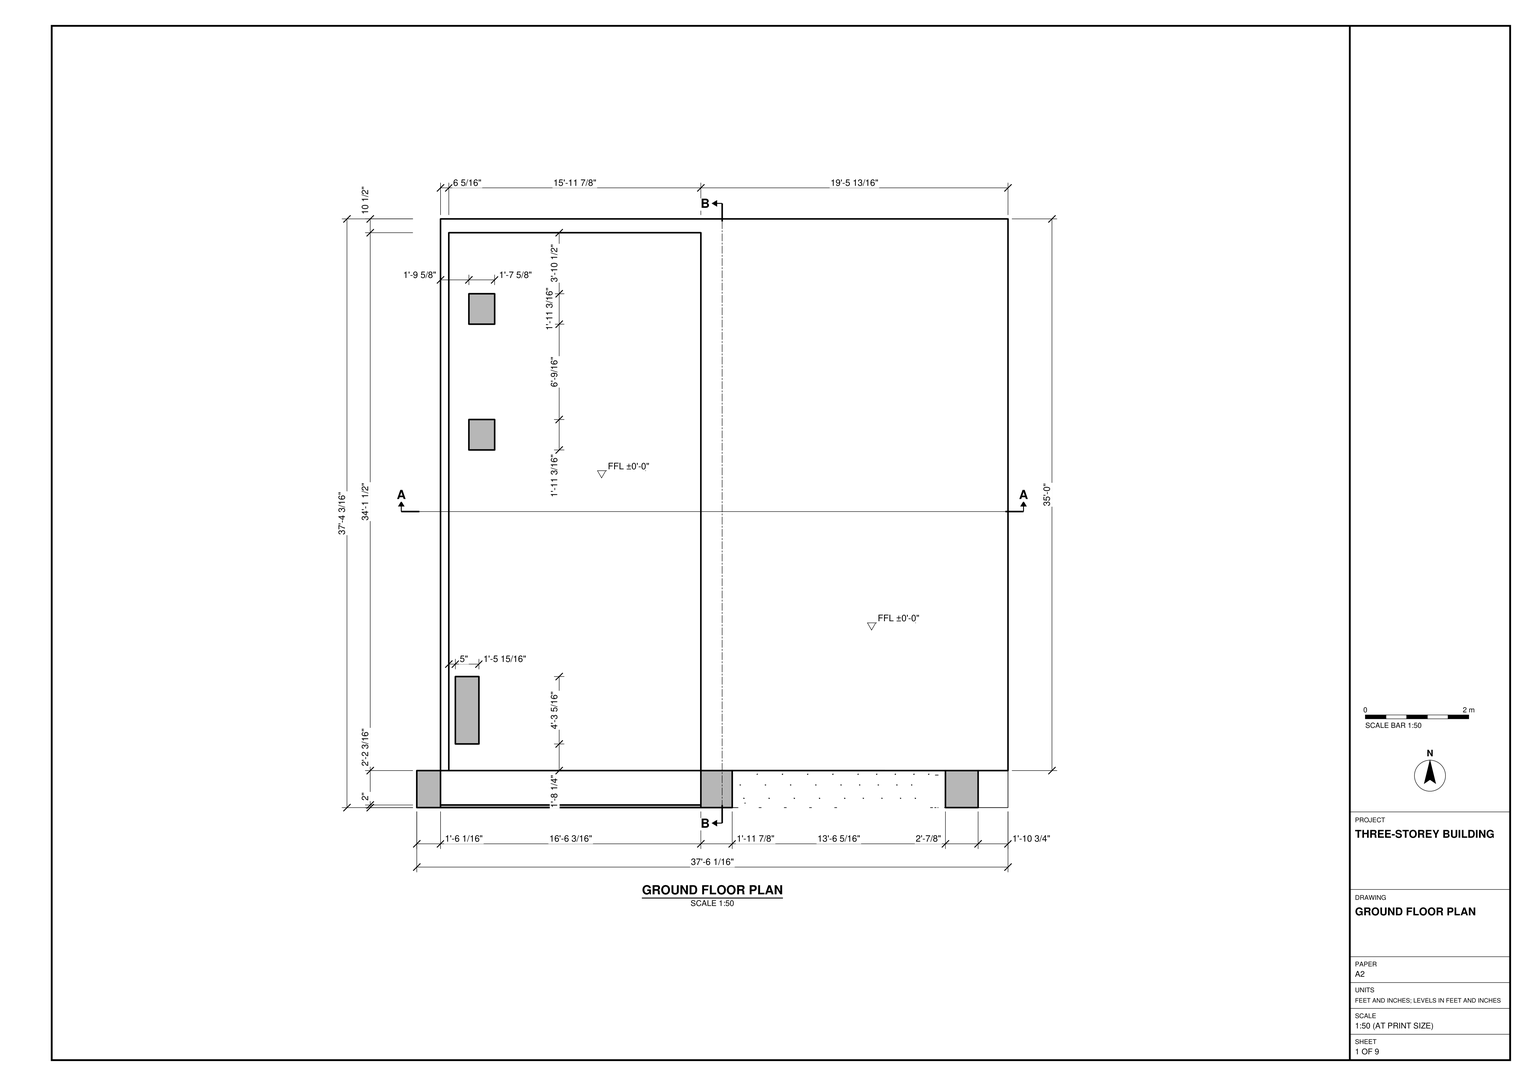
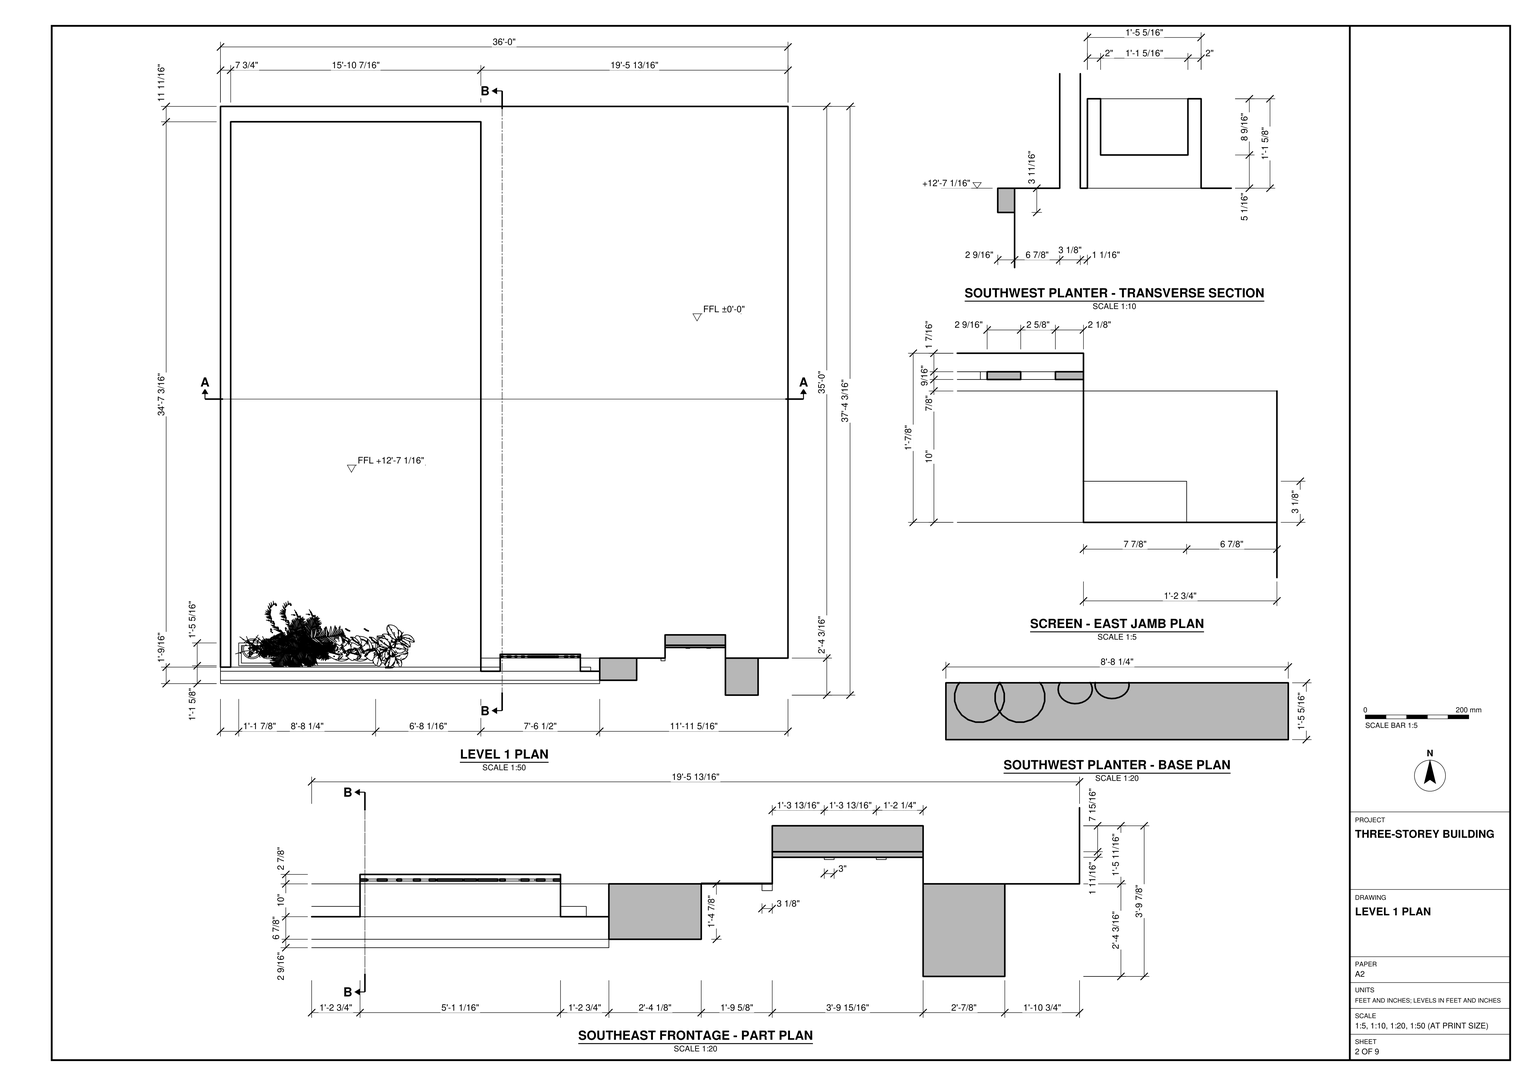
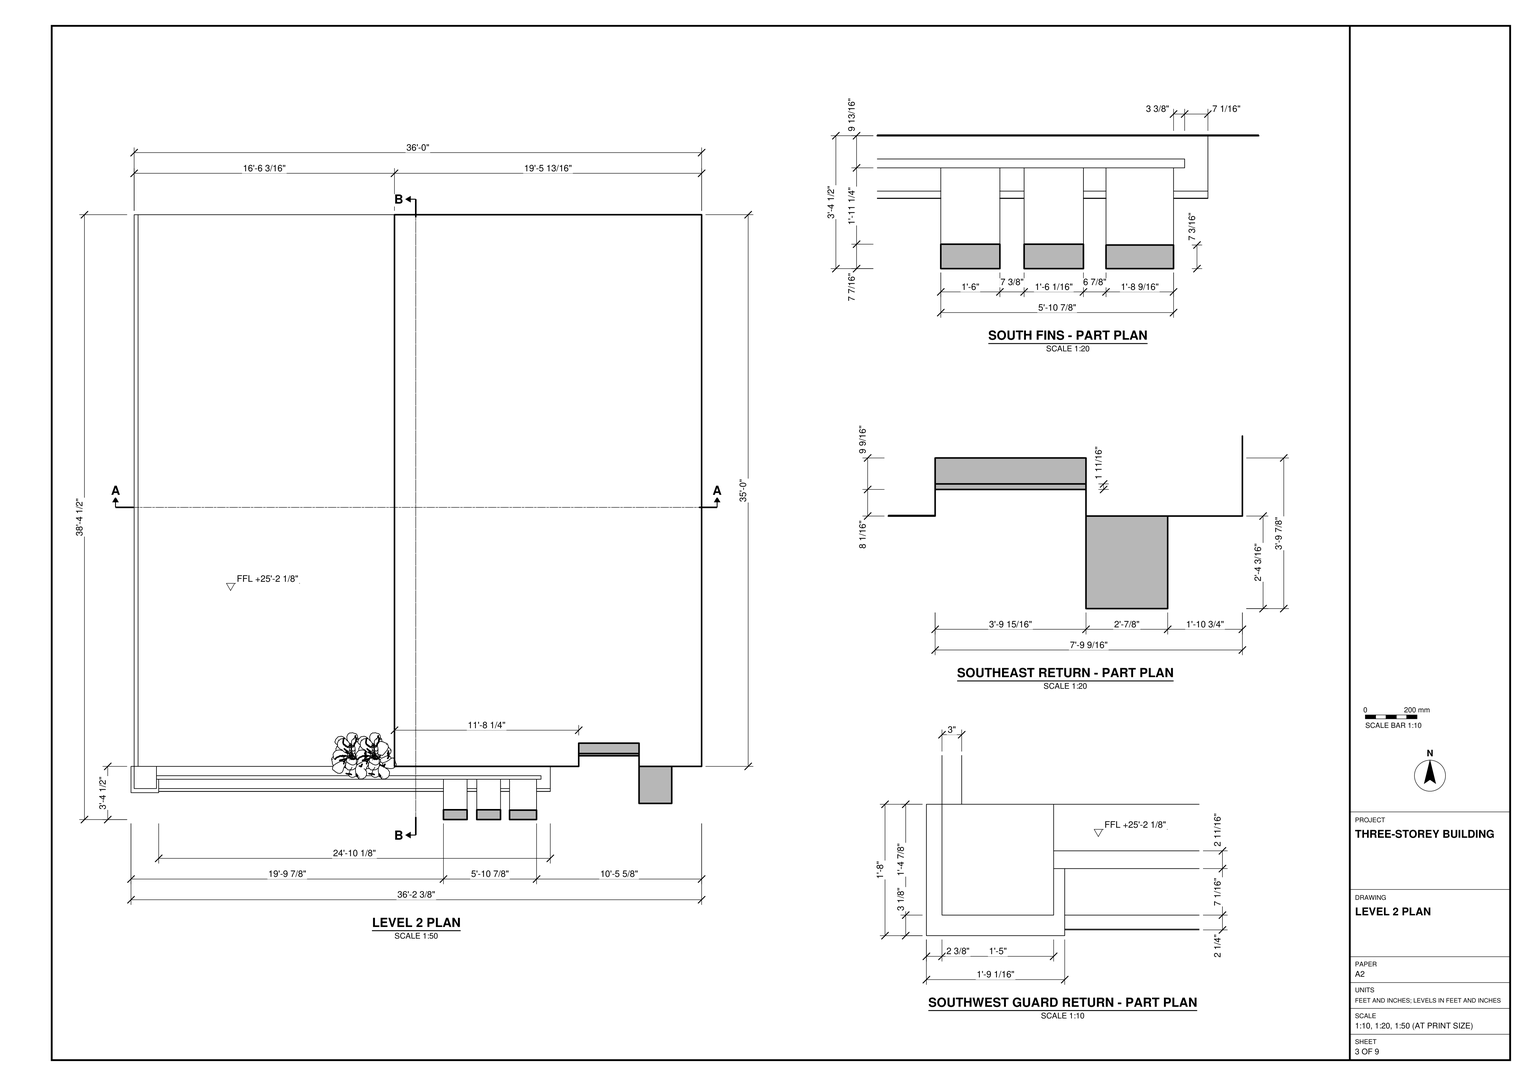
Build the three-storey building in SketchUp from task_files/diagram_01.pdf. Work in feet and inches. The overall model extents, including projections, are 38'-8 15/16" along X, 39'-7 3/8" along Y and 41'-5 7/16" along Z. Set the ground floor at ±0'-0", Level 1 at +12'-7 1/16" and Level 2 at +25'-2 1/8".

Use the plans to lay out the walls at their drawn thicknesses and to locate the supports and openings. Use the sections to establish the slab edges and roof profile. Keep the Level 1 slab over the western bay, leaving the eastern bay open to the ground floor below. Model the south frontage in depth: include the screen and its jamb, the southwest planter, and the recess beside the southeast pier. At Level 2, follow the details for the southwest guard return and the three projecting south fins.

Keep shell elements such as walls, slabs and roof, and each furniture or joinery piece shown, in separate groups or components. Use components for repeated parts. Decor and loose items, including plants, may be any suitable library components. Save one SketchUp model as output_files/three_storey_building_with_a_screened_south_frontage.skp.

# SketchUp Ruby script. Lengths in inches.
U = 1.inch
M = Sketchup.active_model
def pt(a) = Geom::Point3d.new(a.map { |v| v * U })
def face(e, loops, mat)
  f = e.add_face(loops[0].map { |a| pt(a) })
  loops[1..].each { |l| e.add_face(l.map { |a| pt(a) }).erase! }
  f.material = f.back_material = mat if mat
  f
end
# faces: each face lists its corners as indices into pts; further lists are holes
def faces(e, pts, list, mat = nil) = list.each { |f| face(e, (f[0].is_a?(Array) ? f : [f]).map { |l| l.map { |i| pts[i] } }, mat) }
# xy, xz, yz: faces in a plane at the given z, y or x. An outline is a flat list of corners, or four numbers for a rectangle; further outlines are holes
def ring(l) = l.size == 4 ? [[l[0], l[1]], [l[2], l[1]], [l[2], l[3]], [l[0], l[3]]] : l.each_slice(2).to_a
def flat(e, list, mat, &to3) = list.each { |f| face(e, (f[0].is_a?(Array) ? f : [f]).map { |l| ring(l).map { |u, v| to3.(u, v) } }, mat) }
def xy(e, z, list, mat = nil) = flat(e, list, mat) { |x, y| [x, y, z] }
def xz(e, y, list, mat = nil) = flat(e, list, mat) { |x, z| [x, y, z] }
def yz(e, x, list, mat = nil) = flat(e, list, mat) { |y, z| [x, y, z] }
def lines(e, pts, list) = list.each { |a, b| e.add_line(pt(pts[a]), pt(pts[b])) }
# prism: a flat outline (further loops are holes) pulled along v
def prism(e, loops, v, mat = nil)
  f = face(e, loops, mat); d = Geom::Vector3d.new(v.map { |x| x * U })
  f.pushpull(f.normal.samedirection?(d) ? d.length : -d.length)
end
def box(e, o, s, mat = nil) = prism(e, [[o, [o[0] + s[0], o[1], o[2]], [o[0] + s[0], o[1] + s[1], o[2]], [o[0], o[1] + s[1], o[2]]]], [0, 0, s[2]], mat)
def at(x, y, z, deg = 0) = Geom::Transformation.translation(pt([x, y, z])) * Geom::Transformation.rotation(ORIGIN, Z_AXIS, deg.degrees)
def axes(o, x, y, z) = Geom::Transformation.new([*x, 0, *y, 0, *z, 0, *pt(o).to_a, 1])
def part(name) = M.definitions.add(name)
# library, detail: a bought-in or finely detailed component or shape, given as its bounding box
def library(name, o, s) = part(name).tap { |d| box(d.entities, o, s) }
def detail(e, o, s) = box(e.add_group.entities, o, s)
def put(e, d, t, mat = nil) = e.add_instance(d, t).tap { |i| i.material = mat if mat }
def group(e, t, mat = nil) = e.add_group.tap { |g| g.transformation = t; g.material = mat if mat }.entities
root = M.entities
M.materials.add("Generic\#1").color = [131, 113, 113]
M.materials.add("[0136_Charcoal]").color = [35, 35, 35]
M.materials.add("[Color C02]").color = [255, 204, 153]
M.materials.add("[Color C03]").color = [255, 178, 101]
M.materials.add("[Color D03]").color = [255, 216, 101]
M.materials.add("[Color M00]").color = [255, 255, 255]
M.materials.add("[Color M07]").color = [58, 58, 58]
M.materials.add("[Color M08]").color = [30, 30, 30]
M.materials.add("[Translucent Glass Blue]").color = [100, 149, 237]
M.materials["[Translucent Glass Blue]"].alpha = 0.5
M.materials.add("[Translucent Glass Gray]").color = [128, 128, 128]
M.materials["[Translucent Glass Gray]"].alpha = 0.38
M.materials.add("[Wood Bamboo]").color = [177, 105, 43]
M.materials.add("[Wood Cherry Original]").color = [152, 86, 42]
M.materials.add("hymenocallis littoralis").color = [156, 172, 146]
c1 = library("Leaf+Pattern+Wood+Wall+Panel (1)",[0,0,0],[40.87,0.59,87.01])
c2 = library("cvijet+28",[-6.27,-113.67,0],[133.01,125.98,307.58])
c3 = part("Group\#856")
xy(c3.entities,7.38,[[0,0,5.5,15.91]],"hymenocallis littoralis")
p = [[5.5,28.78,0],[5.5,26.79,3.44],[0,26.79,3.44],[0,28.78,0],[0,23.75,6],[5.5,23.75,6],
  [0,15.91,7.38],[5.5,15.91,7.38]]
faces(c3.entities,p,[[0,1,2,3],[4,2,1,5],[6,4,5,7]],"hymenocallis littoralis")
c4 = part("Group\#854")
xy(c4.entities,7.38,[[0,0,5.5,15.91],[0,15.91,5.5,23.87]],"hymenocallis littoralis")
p = [[5.5,31.07,4.3],[5.5,27.74,6.47],[0,27.74,6.47],[0,31.07,4.3],[0,23.87,7.38],[5.5,23.87,7.38]]
faces(c4.entities,p,[[0,1,2,3],[4,2,1,5]],"hymenocallis littoralis")
c5 = part("Group\#857")
xy(c5.entities,7.38,[[0,0,5.6,15.91]],"hymenocallis littoralis")
p = [[5.6,28.78,0],[5.6,26.79,3.44],[0,26.79,3.44],[0,28.78,0],[0,23.75,6],[5.6,23.75,6],
  [0,15.91,7.38],[5.6,15.91,7.38]]
faces(c5.entities,p,[[0,1,2,3],[4,2,1,5],[6,4,5,7]],"hymenocallis littoralis")
c6 = part("Group\#855")
put(c6.entities,c4,axes([6.09,8.57,-0.52],[0.446,0.85617,0.26089],[-0.18444,-0.19731,0.96283],[0.87582,-0.47754,0.0699]))
put(c6.entities,c4,axes([6.29,7.28,-1.71],[0.37058,0.92707,-0.05667],[-0.32382,0.19004,0.99128],[0.87712,-0.32925,0.34964]))
put(c6.entities,c4,axes([11.04,16.14,-0.7],[1,0,0],[0,0.16628,1.02662],[0,-1.18456,0.19186]))
c7 = part("Group\#860")
put(c7.entities,c3,axes([24.57,32.05,-1.76],[0.9552,-0.22102,-0.19681],[0.4036,0.95545,0.88585],[-0.00568,-0.67859,0.7345]))
put(c7.entities,c3,axes([23.95,29.24,-2.4],[0,1,0],[-0.76041,0,0.64945],[0.64945,0,0.76041]))
put(c7.entities,c3,axes([24.22,24.72,-0.48],[-0.70711,0.70711,0],[-0.32757,-0.32757,0.80237],[0.61237,0.61237,0.5]))
put(c7.entities,c4,axes([20.66,37.22,-0.63],[1.12361,0.03262,0.39091],[-0.43499,0.29739,0.78777],[0.09852,-1.27434,0.37535]))
put(c7.entities,c3,axes([28.75,24.45,-2.4],[-1,0,0],[0,-0.76041,0.64945],[0,0.64945,0.76041]))
put(c7.entities,c5,axes([30.4,30.98,-3.7],[0.65676,-0.72002,0.22414],[0.55667,0.66341,0.5],[-0.50871,-0.20361,0.83652]))
put(c7.entities,c5,axes([32.41,29.61,-3.7],[0.04029,-0.97372,0.22414],[0.85287,0.15038,0.5],[-0.52057,0.17102,0.83652]))
put(c7.entities,c3,axes([31.89,25.85,-1.76],[-0.92056,0.33739,-0.19681],[-0.5186,-0.89824,0.88585],[0.08952,0.67268,0.7345]))
put(c7.entities,c3,axes([25.55,34.78,-0.48],[0.86603,0.5,0],[-0.25,0.43301,0.86603],[0.43301,-0.75,0.5]))
put(c7.entities,c5,axes([20.4,16.9375,-8.07],[-0.70711,0.70711,0],[-0.35754,-0.35754,0.65422],[1.3987,1.3987,1.52882]))
put(c7.entities,c3,axes([32.86,34.14,-0.48],[0.76604,-0.64279,0],[0.32139,0.38302,0.86603],[-0.55667,-0.66341,0.5]))
put(c7.entities,c3,axes([27.15,34.7,-0.1],[0.82472,-0.17528,-0.53769],[0.53769,0.53769,0.64945],[0.17528,-0.82472,0.53769]))
put(c7.entities,c3,axes([33.58,28.77,-2.4],[0,-1,0],[0.76041,0,0.64945],[-0.64945,0,0.76041]))
put(c7.entities,c3,axes([26.43,23.87,-2.81],[-0.75126,0.04415,0.65853],[0.53769,-0.53769,0.64945],[0.38276,0.84199,0.3802]))
put(c7.entities,c3,axes([28.78,23.98,-2.4],[-1,0,0],[0,-0.76041,0.64945],[0,0.64945,0.76041]))
put(c7.entities,c3,axes([25.39,25.38,-2.4],[-0.70711,0.70711,0],[-0.53769,-0.53769,0.64945],[0.45923,0.45923,0.76041]))
put(c7.entities,c3,axes([27.32,21.63,-0.1],[-0.45923,0.70711,-0.53769],[-0.76041,0,0.64945],[0.45923,0.70711,0.53769]))
put(c7.entities,c3,axes([25.17,27.625,-1.76],[0.56416,0.80187,-0.19681],[-0.66673,0.66673,0.80532],[0.62659,-0.26057,0.7345]))
put(c7.entities,c5,axes([27.59,27.04,-3.96],[-0.8993,-0.06127,0.43301],[0.2962,-0.8138,0.5],[0.32175,0.57791,0.75]))
put(c7.entities,c5,axes([26.98,24.5,-3.18],[-0.5,0.86603,0],[-0.75,-0.43301,0.5],[0.43301,0.25,0.86603]))
put(c7.entities,c5,axes([24.55,27.74,-3.7],[0.29517,0.92878,0.22414],[-0.85287,0.15038,0.5],[0.43068,-0.33875,0.83652]))
put(c7.entities,c5,axes([24.26,29.8,-3.18],[0.76604,0.64279,0],[-0.47317,0.5639,0.425],[0.32139,-0.38302,0.86603]))
put(c7.entities,c5,axes([25.98,32.46,-3.18],[1,0,0],[0,0.86603,0.5],[0,-0.5,0.86603]))
put(c7.entities,c3,axes([28.78,33.57,-2.4],[1,0,0],[0,0.76041,0.64945],[0,-0.64945,0.76041]))
put(c7.entities,c6,at(14.99,21.38,2.5))
put(c7.entities,c4,axes([34.63,26.34,-1.46],[-0.70089,-0.70877,0.07994],[0.4756,-0.38088,0.79293],[-0.53156,0.59378,0.60405]))
put(c7.entities,c4,axes([28.14,16.92,1.8125],[-1.19719,0.6912,0],[-0.09607,-0.16641,0.94244],[0.68444,1.18549,0.17613]))
put(c7.entities,c4,axes([31.5625,35.84,0.97],[0.66765,-1.1564,0.35779],[0.04445,0.30732,0.91033],[-1.20828,-0.64496,0.17012]))
put(c7.entities,c4,axes([38.94,22.51,0.89],[-0.97932,-0.67164,-0.05202],[0.27787,-0.41401,0.90999],[-0.85985,0.93577,0.32097]))
put(c7.entities,c4,axes([38.44,21.09,1.98],[-1.02864,-0.54856,0.2395],[0.33481,0.06999,0.88388],[-0.77261,1.08328,0.06417]))
put(c7.entities,c5,axes([35.02,30.51,-1.3],[-0.17365,-0.98481,0],[0.60224,-0.10619,0.79122],[-0.7792,0.13739,0.61153]))
put(c7.entities,c5,axes([29.41,22.33,-1.3],[-0.93969,0.34202,0],[-0.20915,-0.57465,0.79122],[0.27061,0.74351,0.61153]))
put(c7.entities,c4,axes([19.64,36,-1.62],[1.18194,0.09546,0.08234],[-0.14377,0.68823,0.76313],[0.21457,-1.1326,0.62386]))
put(c7.entities,c5,axes([24.25,24.14,-1.3],[-0.34202,0.93969,0],[-0.57465,-0.20915,0.79122],[0.74351,0.27061,0.61153]))
put(c7.entities,c5,axes([25.98,34.61,-1.3],[1,0,0],[0,0.61153,0.79122],[0,-0.79122,0.61153]))
put(c7.entities,c5,axes([31.16,34.41,-1.64],[0.56518,-0.80224,-0.19234],[0.73413,0.34233,0.72935],[-0.47639,-0.50772,0.71782]))
put(c7.entities,c5,axes([40.52,26.84,-5.82],[-0.42262,-0.90631,0],[0.48019,-0.22391,0.68552],[-1.43418,0.66877,1.22305]))
put(c7.entities,c3,axes([29.86,38.42,-1.01],[0.89064,-0.37013,0.26413],[-0.03924,0.63286,1.01918],[-0.45353,-0.76487,0.45748]))
put(c7.entities,c3,axes([29.34,22.4,-0.48],[-0.99619,-0.08716,0],[0.04358,-0.4981,0.86603],[-0.07548,0.86273,0.5]))
c8 = part("Group\#858")
xz(c8.entities,10.07,[[9.07,0,10.07,31.01],[0,31.01,0,45.12,20.13,45.12,20.13,31.01,10.07,31.01,10.07,32.58,9.07,32.58,9.07,31.01]],"hymenocallis littoralis")
yz(c8.entities,10.07,[[0,31.01,20.13,45.12]],"hymenocallis littoralis")
p = [[9.57,9.2,0],[10.07,10.07,0],[10.07,10.07,31.01],[10.07,10.07,32.58],[9.57,9.2,32.58]]
faces(c8.entities,p,[[0,1,2,3,4]],"hymenocallis littoralis")
c9 = part("cây lá nắng")
put(c9.entities,c7,axes([49.26,-2.75,0],[0.63109,0.63109,0],[-0.63109,0.63109,0],[0,0,0.935]))
g1 = group(c9.entities,at(26.6,-8.68,0))
put(g1,c3,axes([-4.72,35.73,-1.65],[0.74231,0.46334,-0.18402],[-0.34827,0.85768,0.82827],[0.42467,-0.43184,0.68675]))
put(g1,c3,axes([-3.34,33.57,-2.24],[-0.63109,0.63109,0],[-0.47989,-0.47989,0.60723],[0.40986,0.40986,0.71098]))
put(g1,c3,axes([-0.3125,30.89,-0.45],[-0.8925,0,0],[0,-0.41345,0.75022],[0,0.77293,0.4675]))
put(g1,c4,axes([-10.79,39.66,-0.59],[0.68852,0.72969,0.3655],[-0.4622,-0.08684,0.73657],[0.86641,-0.74205,0.35095]))
put(g1,c3,axes([2.71,33.57,-2.24],[-0.63109,-0.63109,0],[0.47989,-0.47989,0.60723],[-0.40986,0.40986,0.71098]))
put(g1,c5,axes([-0.37,38.74,-3.46],[0.86887,-0.03992,0.20957],[-0.06737,0.76999,0.4675],[-0.19255,-0.44954,0.78214]))
put(g1,c5,axes([1.76,39.14,-3.46],[0.63993,-0.58908,0.20957],[0.44333,0.63315,0.4675],[-0.43646,-0.2206,0.78214]))
put(g1,c3,axes([3.81,36.4375,-1.65],[-0.79389,-0.36803,-0.18402],[0.23959,-0.89415,0.82827],[-0.36803,0.48102,0.68675]))
put(g1,c3,axes([-5.83,38.07,-0.45],[0.231,0.86209,0],[-0.43104,0.1155,0.80973],[0.74659,-0.20005,0.4675]))
put(g1,c5,axes([2.18,23.5625,-7.55],[-0.8925,0,0],[0,-0.45128,0.6117],[0,1.76542,1.42944]))
put(g1,c3,axes([-0.8125,42.28,-0.45],[0.8891,0.07779,0],[-0.03889,0.44455,0.80973],[0.06737,-0.76999,0.4675]))
put(g1,c3,axes([-4.76,39.03,-0.09],[0.63109,0.40986,-0.50274],[0,0.67866,0.60723],[0.63109,-0.40986,0.50274]))
put(g1,c3,axes([3.03,39.35,-2.24],[0.63109,-0.63109,0],[0.47989,0.47989,0.60723],[-0.40986,-0.40986,0.71098]))
put(g1,c3,axes([1.61,31.74,-2.625],[-0.50198,-0.44625,0.61573],[0.67866,0,0.60723],[-0.28982,0.77293,0.35549]))
put(g1,c3,axes([3.03,33.3,-2.24],[-0.63109,-0.63109,0],[0.47989,-0.47989,0.60723],[-0.40986,0.40986,0.71098]))
put(g1,c3,axes([0.01,32.04,-2.24],[-0.8925,0,0],[0,-0.67866,0.60723],[0,0.57963,0.71098]))
put(g1,c3,axes([3.59,30.89,-0.09],[-0.73607,0.15643,-0.50274],[-0.47989,-0.47989,0.60723],[-0.15643,0.73607,0.50274]))
put(g1,c3,axes([-1.55,33.32,-1.65],[-0.15002,0.86209,-0.18402],[-0.84154,0,0.75297],[0.55988,0.231,0.68675]))
put(g1,c5,axes([0.35,34.48,-3.71],[-0.52887,-0.60621,0.40487],[0.70051,-0.32665,0.4675],[-0.16166,0.56777,0.70125]))
put(g1,c5,axes([2.61,39.13,-1.74],[-0.86209,0.231,0],[-0.23031,-0.85954,0.15531],[0.03162,0.11799,0.91645]))
put(g1,c5,axes([-2.02,33,-3.46],[-0.39986,0.77243,0.20957],[-0.63315,-0.44333,0.4675],[0.48558,0.05802,0.78214]))
put(g1,c5,axes([-3.49,34.12,-2.97],[0.07779,0.8891,0],[-0.65449,0.05726,0.39737],[0.44455,-0.03889,0.80973]))
put(g1,c5,axes([-4.09,36.88,-2.97],[0.63109,0.63109,0],[-0.54654,0.54654,0.4675],[0.31555,-0.31555,0.80973]))
put(g1,c3,axes([-3.02,39.35,-2.24],[0.63109,0.63109,0],[-0.47989,0.47989,0.60723],[0.40986,-0.40986,0.71098]))
put(g1,c6,axes([-4.03,22.95,2.33],[0.63109,0.63109,0],[-0.63109,0.63109,0],[0,0,0.935]))
put(g1,c4,axes([5.24,38.48,-1.37],[0.00497,-0.88963,0.07474],[0.54052,0.05978,0.74139],[-0.71019,0.03927,0.56479]))
put(g1,c4,axes([7.08,28.4375,1.7],[-1.19175,-0.31933,0],[0.04439,-0.16565,0.88118],[-0.31621,1.1801,0.16468]))
put(g1,c4,axes([-2.7,42.54,0.91],[1.15114,-0.30845,0.33454],[-0.1659,0.22199,0.85115],[-0.3555,-1.16957,0.15907]))
put(g1,c4,axes([10.37,38.78,0.83],[-0.19417,-1.04191,-0.04864],[0.43664,-0.08592,0.85084],[-1.1332,0.04791,0.30011]))
put(g1,c4,axes([10.95,37.5625,1.85],[-0.30298,-0.99536,0.22393],[0.16713,0.25547,0.82643],[-1.17124,0.19607,0.06]))
put(g1,c5,axes([2.84,41.36,-1.22],[0.51192,-0.73109,0],[0.44708,0.31305,0.73979],[-0.57846,-0.40504,0.57178]))
put(g1,c5,axes([4.47,32.65,-1.22],[-0.80888,-0.37719,0],[0.23066,-0.49465,0.73979],[-0.29844,0.64,0.57178]))
put(g1,c4,axes([-10.32,35.12,-1.51],[0.68567,0.80616,0.07699],[-0.52507,0.3436,0.71352],[0.85019,-0.57936,0.58331]))
put(g1,c5,axes([0.07,30.54,-1.22],[-0.80888,0.37719,0],[-0.23066,-0.49465,0.73979],[0.29844,0.64,0.57178]))
put(g1,c5,axes([-5.45,38.24,-1.22],[0.63109,0.63109,0],[-0.38593,0.38593,0.73979],[0.49934,-0.49934,0.57178]))
put(g1,c5,axes([-2.05,41.38,-1.53],[0.86296,-0.14961,-0.17984],[0.24726,0.67935,0.68194],[0.01977,-0.62107,0.67116]))
put(g1,c5,axes([8.63,42.51,-5.4375],[0.30525,-0.83868,0],[0.44435,0.16173,0.64096],[-1.32716,-0.48305,1.14356]))
put(g1,c3,axes([-5.4,43.09,-0.94],[0.79566,0.32849,0.24696],[-0.42416,0.37462,0.95293],[0.19648,-0.76892,0.42774]))
put(g1,c3,axes([4.38,32.65,-0.45],[-0.57369,-0.68369,0],[0.34185,-0.28684,0.80973],[-0.5921,0.49683,0.4675]))
put(g1,c5,axes([-2,33.84,-0.15],[-0.24601,0.85793,0],[-0.85539,-0.24528,0.15531],[0.11742,0.03367,0.91645]))
put(g1,c5,axes([0.17,30.83,-4.47],[-0.24601,0.85793,0],[-0.85539,-0.24528,0.15531],[0.11742,0.03367,0.91645]))
put(g1,c5,axes([-1.97,32.18,-4.47],[0.58524,0.67383,0],[-0.67184,0.58351,0.15531],[0.09222,-0.0801,0.91645]))
put(g1,c5,axes([-2,34.71,-4.47],[0.88392,-0.12346,0],[0.12309,0.88131,0.15531],[-0.0169,-0.12098,0.91645]))
put(g1,c5,axes([0.11,36.12,-4.47],[0.37822,-0.8084,0],[0.80601,0.37711,0.15531],[-0.11064,-0.05177,0.91645]))
put(c9.entities,c8,axes([29.71,14.29,6.94],[0.425,0.73612,0],[-0.6771,0.39092,-0.33349],[-0.26859,0.15507,0.72712]))
put(c9.entities,c8,axes([42.0625,26.12,6.94],[0.85,0,0],[0,0.78185,-0.33349],[0,0.33349,0.78185]))
put(c9.entities,c7,axes([7.3125,23.0625,0],[0.8925,0,0],[0,0.8925,0],[0,0,0.935]))
put(c9.entities,c8,axes([24.4375,40.23,2.05],[0.85,0,0],[0,0.85,0],[0,0,0.85]))
c10 = part("Planting+101")
put(c10.entities,c9,axes([21.34,32.96,-4.59],[0,-0.71,0],[-0.71,0,0],[0,0,0.71]))
c11 = library("Flora+17",[-57.52,158.6,-38.64],[66.99,62.88,77.28])
c12 = library("Group_2",[-1.28,-0.39,0],[21.22,20.51,48.44])
c13 = library("Plant+2 (1)",[-9.13,-9.52,0],[51.76,51.77,66.88])
xy(root,-18.8125,[[0,12.29,18.0625,40.48],[18.0625,12.29,450.0625,40.48],[18.0625,40.48,450.0625,460.48]])
xy(root,-1.3125,[[243.55,15.72,399.01,37.05]])
xy(root,0,[[18.0625,12.29,216.25,40.48],[240.125,12.29,402.4375,40.48],[402.4375,12.29,427.3125,40.48],[427.3125,12.29,450.0625,40.48],[18.0625,40.48,24.375,40.48,24.375,449.98,216.25,449.98,216.25,40.48,450.0625,40.48,450.0625,460.48,18.0625,460.48],
  [[24.375,40.48,216.25,449.98],[29.35,60.76,47.29,112.07],[39.66,284.5625,59.28,307.75],[39.66,380.32,59.28,403.5]]])
xy(root,15.5,[[[240.125,12.29,402.4375,40.48],[243.55,15.72,399.01,37.05]]])
xy(root,35.04,[[216.25,40.48,356.5,40.78]])
xy(root,35.34,[[216.25,40.48,356.5,40.78]])
xy(root,62.8125,[[0,12.29,18.0625,40.48],[216.25,12.29,240.125,40.48]])
xy(root,64.875,[[356.5,38.1,356.5,38.41,353.38,38.41,353.38,40.48,402.4375,40.48,402.4375,38.1]],"[Color M00]")
xy(root,68.125,[[356.5,40.48,402.4375,40.48,402.4375,49.32,391.1875,49.32,391.1875,47.88,388.1875,47.88,388.1875,49.32,375.35,49.32,375.35,47.88,372.35,47.88,372.35,49.32,356.5,49.32],[372.35,47.88,372.35,49.32,356.5,49.32,356.5,50.26,402.4375,50.26,402.4375,49.32,391.1875,49.32,391.1875,47.88,388.1875,47.88,388.1875,49.32,375.35,49.32,375.35,47.88],[356.5,50.26,402.4375,58.16]])
xy(root,68.125,[[356.5,38.1,402.4375,40.48]],"[Color M00]")
xy(root,68.39,[[216.25,40.48,356.5,40.78]])
xy(root,68.69,[[216.25,40.48,356.5,40.78]])
xy(root,69.4375,[[0,12.29,18.0625,40.48],[216.25,12.29,240.125,40.48]])
xy(root,120,[[18.0625,21.04,334.88,23.6],[18.0625,23.6,334.88,40.48]])
xy(root,120,[[[24.375,40.48,216.25,449.98],[29.35,60.76,47.29,112.07],[39.66,380.32,59.28,403.5],[39.66,284.5625,59.28,307.75]]],"[Color C02]")
xy(root,123.875,[[18.0625,21.04,334.88,23.6]],"[Color M07]")
xy(root,135.09,[[334.88,40.48,353.38,40.78]])
xy(root,135.39,[[334.88,40.48,353.38,40.78]])
xy(root,138.875,[[372.35,47.88,375.35,48.57],[388.1875,47.88,391.1875,48.57],[356.5,48.57,372.35,49.32],[375.35,48.57,388.1875,49.32],[391.1875,48.57,402.4375,49.32]])
xy(root,147.375,[[18.0625,21.04,306.75,23.6]])
xy(root,151.0625,[[18.0625,23.6,306.75,30.47],[216.25,30.47,299.88,33.6],[299.88,30.47,306.75,30.47,306.75,40.48,216.25,40.48,216.25,33.6,299.88,33.6]])
xy(root,151.0625,[[[25.8125,33.6,216.25,448.79],[31.93,34.6875,136.18,52]]],"[Color C02]")
xy(root,151.0625,[[18.0625,21.04,306.75,23.6]],"[Color M07]")
xy(root,156.125,[[33.94,36.69,134.18,49.99]])
xy(root,164.6875,[[[31.93,34.6875,136.18,52],[33.94,36.69,134.18,49.99]]])
xy(root,165.79,[[230.98,30.47,292.03,43.35]])
xy(root,168.43,[[334.88,40.48,356.5,40.78]])
xy(root,168.43,[[353.38,38.41,356.5,40.48]],"[Wood Bamboo]")
xy(root,168.73,[[334.88,40.48,356.5,40.78]])
xy(root,193.5,[[18.0625,30.47,216.25,33.6]])
xy(root,196.5,[[18.0625,30.47,216.25,33.6]],"[Color M07]")
xy(root,201.78,[[334.88,40.48,356.5,40.78]])
xy(root,202.08,[[334.88,40.48,356.5,40.78]])
xy(root,204.3125,[[15.125,28.79,25.8125,33.6],[25.8125,28.79,30.625,150.91],[15.125,33.6,18.0625,150.91],[18.0625,33.6,25.8125,150.91]])
xy(root,207.6875,[[15.125,28.79,30.625,150.91]],"Generic\#1")
xy(root,235.13,[[334.88,40.48,356.5,40.78]])
xy(root,235.43,[[334.88,40.48,356.5,40.78]])
xy(root,256.34,[[230.98,30.47,292.03,43.35]])
xy(root,268.48,[[334.88,40.48,356.5,40.78]])
xy(root,268.78,[[334.88,40.48,356.5,40.78]])
xy(root,271.0625,[[18.0625,21.48,18.0625,40.48,216.25,40.48,216.25,30.47,306.75,30.47,306.75,21.48],[216.25,30.47,306.75,40.48]])
xy(root,271.0625,[[18.0625,40.48,18.0625,150.91,25.8125,150.91,25.8125,448.79,216.25,448.79,216.25,40.48]],"[Color C02]")
xy(root,274.625,[[18.0625,21.48,306.75,23.6]],"[Color M07]")
xy(root,298.5625,[[18.0625,21.35,334.88,21.48],[18.0625,21.48,334.88,23.6]])
xy(root,301.82,[[334.88,40.48,356.5,40.78]])
xy(root,302.0625,[[18.0625,23.6,35.06,40.48]])
xy(root,302.125,[[18.0625,21.35,334.88,21.48],[18.0625,21.48,334.88,23.6],[35.06,23.6,334.88,23.6,334.88,40.48,35.06,40.48,35.06,33.39,327.79,33.39,327.79,30.6875,35.06,30.6875],[18.0625,40.48,21.0625,460.48],[21.0625,40.48,216.25,460.48],
  [334.88,40.48,356.5,40.78]])
xy(root,315.16,[[253.53,0,271.53,30.6875],[278.91,0,296.97,30.6875],[303.85,0,324.41,30.6875]])
xy(root,333.25,[[18.0625,40.48,21.0625,460.48]])
xy(root,333.3125,[[15.6875,20.48,15.6875,40.48,18.0625,40.48,18.0625,23.6,35.06,23.6,35.06,30.6875,36.75,30.6875,36.75,20.48]],"[Color M07]")
xy(root,334.8125,[[35.06,30.6875,327.79,33.39]])
xy(root,335.17,[[216.25,40.48,356.5,40.78]])
xy(root,335.47,[[216.25,40.48,356.5,40.78]])
xy(root,336.9375,[[18.0625,23.6,35.06,40.48],[18.0625,40.48,21.0625,460.48]])
xy(root,336.9375,[[303.85,7.1875,324.41,30.6875],[253.53,7.4375,271.53,30.6875],[278.91,7.4375,296.97,30.6875]],"Generic\#1")
xy(root,336.9375,[[15.6875,20.48,36.75,20.48,36.75,30.6875,35.06,30.6875,35.06,23.6,18.0625,23.6,18.0625,40.48,15.6875,40.48],[35.06,30.6875,327.79,33.39]],"[Color M07]")
xy(root,368.52,[[216.25,40.48,356.5,40.78]])
xy(root,368.82,[[216.25,40.48,356.5,40.78]])
xy(root,391.0625,[[119.5,12.29,402.4375,40.48],[356.5,40.48,402.4375,48.57],[356.5,48.57,402.4375,50.26],[356.5,50.26,402.4375,58.16]])
xy(root,391.0625,[[119.5,40.48,216.25,460.48]],"[Color C02]")
xy(root,391.0625,[[119.5,6.98,402.4375,12.29]],"[Color M07]")
xy(root,394.0625,[[119.5,6.98,402.4375,12.29]],"[Color M07]")
xy(root,418.375,[[119.5,6.98,427.3125,12.29]],"[Color M07]")
xy(root,422.125,[[119.5,12.29,427.3125,40.48],[119.5,40.48,234.77,460.48]])
xy(root,422.125,[[119.5,6.98,427.3125,12.29]],"[Color M07]")
xy(root,425.3125,[[253.53,7.4375,271.53,40.48],[278.91,7.4375,296.97,40.48]])
xy(root,425.375,[[303.85,7.1875,324.41,40.48]])
xy(root,436.625,[[278.91,0,296.97,40.48],[303.85,0,324.41,40.48]])
xy(root,436.625,[[253.53,0,271.53,40.48]],"Generic\#1")
xy(root,457.3125,[[217.52,25.6,234.77,475.35],[234.77,25.6,464.9375,40.48],[234.77,40.48,450.0625,460.48],[450.0625,40.48,464.9375,475.35],[234.77,460.48,450.0625,475.35]])
xy(root,457.3125,[[217.52,19.98,234.77,25.6],[234.77,19.98,464.9375,25.6]],"[Color M07]")
xy(root,460.3125,[[217.52,19.98,234.77,25.6],[234.77,19.98,464.9375,25.6]],"[Color M07]")
xy(root,475.3125,[[217.52,19.98,464.9375,25.6]],"[Color M07]")
xy(root,478.625,[[217.52,25.6,464.9375,475.35]])
xy(root,478.625,[[217.52,19.98,464.9375,25.6]],"[Color M07]")
xz(root,0,[[253.53,315.16,271.53,436.625],[278.91,315.16,296.97,436.625],[303.85,315.16,324.41,436.625]],"Generic\#1")
xz(root,6.98,[[119.5,391.0625,402.4375,394.0625],[119.5,418.375,427.3125,422.125]],"[Color M07]")
xz(root,7.1875,[[303.85,336.9375,324.41,425.375]])
xz(root,7.4375,[[278.91,334.8125,296.97,336.9375],[253.53,336.9375,271.53,425.3125],[278.91,336.9375,296.97,425.3125]])
xz(root,12.29,[[0,-18.8125,18.0625,62.8125],[18.0625,-18.8125,450.0625,-18.8125,450.0625,0,240.125,0,240.125,62.8125,216.25,62.8125,216.25,0,18.0625,0],[402.4375,0,427.3125,0,427.3125,418.375,119.5,418.375,119.5,394.0625,402.4375,394.0625],[0,62.8125,18.0625,69.4375],[216.25,62.8125,240.125,69.4375],
  [119.5,391.0625,402.4375,394.0625],[119.5,418.375,427.3125,422.125]])
xz(root,12.29,[[240.125,0,402.4375,15.5]],"Generic\#1")
xz(root,15.72,[[243.55,-1.3125,399.01,15.5]])
xz(root,19.98,[[217.52,457.3125,464.9375,460.3125],[217.52,475.3125,464.9375,478.625]],"[Color M07]")
xz(root,20.48,[[15.6875,333.3125,36.75,336.9375]],"[Color M07]")
xz(root,21.04,[[18.0625,120,334.88,123.875],[18.0625,147.375,306.75,151.0625]],"[Color M07]")
xz(root,21.35,[[18.0625,298.5625,334.88,302.125]],"[Color M07]")
xz(root,21.48,[[18.0625,298.5625,334.88,302.125]])
xz(root,21.48,[[18.0625,271.0625,306.75,274.625]],"[Color M07]")
xz(root,23.6,[[18.0625,120,334.88,123.875],[18.0625,123.875,334.88,123.875,334.88,298.5625,18.0625,298.5625,18.0625,274.625,306.75,274.625,306.75,147.375,18.0625,147.375],[18.0625,147.375,306.75,151.0625],[18.0625,298.5625,18.0625,302.0625,35.06,302.0625,35.06,302.125,334.88,302.125,334.88,298.5625],[18.0625,302.0625,35.06,302.125],
  [18.0625,302.125,35.06,333.3125],[18.0625,333.3125,35.06,336.9375]])
xz(root,25.6,[[217.52,457.3125,464.9375,460.3125],[217.52,460.3125,464.9375,475.3125],[217.52,475.3125,464.9375,478.625]])
xz(root,28.79,[[15.125,204.3125,30.625,207.6875]],"Generic\#1")
xz(root,30.47,[[[216.25,151.0625,306.75,271.0625],[230.98,165.79,292.03,256.34]]])
xz(root,30.47,[[18.0625,193.5,216.25,196.5]],"[Color M07]")
xz(root,30.47,[[18.0625,151.0625,216.25,193.5]],"[Translucent Glass Gray]")
xz(root,30.6875,[[253.53,315.16,271.53,334.8125],[35.06,334.8125,36.75,336.9375],[253.53,334.8125,271.53,336.9375],[271.53,334.8125,278.91,336.9375],[278.91,334.8125,296.97,336.9375],
  [296.97,334.8125,303.85,336.9375],[303.85,334.8125,324.41,336.9375],[324.41,334.8125,327.79,336.9375]])
xz(root,30.6875,[[36.75,334.8125,253.53,336.9375]],"[Color M07]")
xz(root,30.6875,[[35.06,302.125,327.79,302.125,327.79,334.8125,324.41,334.8125,324.41,315.16,303.85,315.16,303.85,334.8125,296.97,334.8125,296.97,315.16,278.91,315.16,278.91,334.8125,271.53,334.8125,271.53,315.16,253.53,315.16,253.53,334.8125,36.75,334.8125,36.75,333.3125,35.06,333.3125],[35.06,333.3125,36.75,334.8125]],"[Translucent Glass Gray]")
xz(root,33.39,[[35.06,334.8125,327.79,336.9375]],"[Color M07]")
xz(root,33.39,[[35.06,302.125,327.79,334.8125]],"[Translucent Glass Gray]")
xz(root,33.6,[[18.0625,151.0625,25.8125,193.5],[18.0625,193.5,25.8125,196.5],[25.8125,193.5,216.25,196.5]])
xz(root,33.6,[[18.0625,196.5,25.8125,204.3125]],"Generic\#1")
xz(root,33.6,[[25.8125,151.0625,216.25,193.5]],"[Translucent Glass Gray]")
xz(root,34.6875,[[31.93,151.0625,136.18,164.6875]])
xz(root,36.69,[[33.94,156.125,134.18,164.6875]])
xz(root,37.05,[[243.55,-1.3125,356.5,15.5],[356.5,-1.3125,399.01,15.5]])
xz(root,38.1,[[356.5,64.875,402.4375,68.125]],"[Color M00]")
xz(root,38.41,[[353.38,64.875,356.5,168.43]],"[Color M00]")
xz(root,40.48,[[0,-18.8125,18.0625,55.8125],[18.0625,-18.8125,450.0625,0],[24.375,0,216.25,120],[216.25,0,240.125,35.04],[240.125,0,402.4375,15.5],
  [402.4375,0,427.3125,120],[216.25,35.04,240.125,35.34],[216.25,35.34,240.125,55.8125],[0,55.8125,18.0625,62.8125],[216.25,55.8125,240.125,62.8125],
  [0,62.8125,18.0625,69.4375],[216.25,62.8125,240.125,68.39],[216.25,68.39,240.125,68.69],[216.25,68.69,240.125,69.4375],[216.25,101.74,353.38,102.04],
  [402.4375,120,427.3125,151.0625],[306.75,151.0625,334.88,168.73],[402.4375,151.0625,427.3125,271.0625],[306.75,168.73,334.88,202.08],[306.75,202.08,334.88,235.43],
  [306.75,235.43,334.88,268.78],[306.75,268.78,334.88,271.0625],[18.0625,271.0625,18.0625,302.0625,35.06,302.0625,35.06,302.125,334.88,302.125,334.88,271.0625],[402.4375,271.0625,427.3125,302.125],[18.0625,302.0625,35.06,302.125],
  [18.0625,302.125,21.0625,333.25],[21.0625,302.125,35.06,336.9375],[402.4375,302.125,427.3125,391.0625],[18.0625,333.25,21.0625,336.9375],[15.6875,333.3125,18.0625,336.9375],
  [119.5,391.0625,427.3125,422.125]])
xz(root,40.48,[[18.0625,0,24.375,120],[[427.3125,0,450.0625,0,450.0625,457.3125,234.77,457.3125,234.77,422.125,427.3125,422.125],[303.85,425.375,324.41,436.625],[278.91,425.3125,296.97,436.625],[253.53,425.3125,271.53,436.625]]],"Generic\#1")
xz(root,40.48,[[240.125,15.5,356.5,35.04],[356.5,15.5,402.4375,64.875],[240.125,35.34,356.5,35.34,356.5,64.875,353.38,64.875,353.38,68.39,240.125,68.39],[353.38,64.875,356.5,68.39],[356.5,64.875,402.4375,68.125],
  [353.38,68.39,356.5,68.69],[240.125,68.69,353.38,68.69,353.38,101.74,216.25,101.74,216.25,69.4375,240.125,69.4375],[353.38,68.69,356.5,101.74],[216.25,102.04,353.38,102.04,353.38,135.09,334.88,135.09,334.88,120,216.25,120],[353.38,102.04,356.5,135.09],
  [334.88,135.39,353.38,168.43],[353.38,135.39,356.5,168.43],[334.88,168.73,356.5,201.78],[334.88,202.08,356.5,235.13],[334.88,235.43,356.5,268.48],
  [334.88,268.78,356.5,301.82],[216.25,302.125,356.5,335.17],[216.25,335.47,356.5,368.52],[216.25,368.82,356.5,391.0625]],"[Wood Bamboo]")
xz(root,40.78,[[216.25,35.04,356.5,35.34],[216.25,68.39,356.5,68.69],[334.88,135.09,353.38,135.39],[334.88,168.43,356.5,168.73],[334.88,201.78,356.5,202.08],
  [334.88,235.13,356.5,235.43],[334.88,268.48,356.5,268.78],[334.88,301.82,356.5,302.125],[216.25,335.17,356.5,335.47],[216.25,368.52,356.5,368.82]])
xz(root,43.35,[[230.98,165.79,292.03,256.34]])
xz(root,47.88,[[372.35,68.125,375.35,138.875],[388.1875,68.125,391.1875,138.875]],"[Color M07]")
xz(root,48.57,[[356.5,138.875,402.4375,144.875],[356.5,185.625,402.4375,188.625],[356.5,321.0625,402.4375,324.0625],[356.5,354.5625,402.4375,357.5625]],"[Color M07]")
xz(root,48.57,[[356.5,144.875,402.4375,185.625],[356.5,188.625,402.4375,321.0625],[356.5,324.0625,402.4375,354.5625],[356.5,357.5625,402.4375,391.0625]],"[Translucent Glass Blue]")
xz(root,49.32,[[356.5,68.125,372.35,138.875],[375.35,68.125,388.1875,138.875],[391.1875,68.125,402.4375,138.875]],"[0136_Charcoal]")
xz(root,49.99,[[33.94,156.125,134.18,164.6875]])
xz(root,50.26,[[356.5,68.125,402.4375,391.0625]])
xz(root,52,[[31.93,151.0625,136.18,164.6875]])
xz(root,58.16,[[356.5,68.125,402.4375,391.0625]])
xz(root,60.76,[[29.35,0,47.29,120]],"Generic\#1")
xz(root,112.07,[[29.35,0,47.29,120]])
xz(root,150.91,[[15.125,204.3125,18.0625,207.6875],[18.0625,204.3125,25.8125,207.6875],[25.8125,204.3125,30.625,207.6875]])
xz(root,150.91,[[18.0625,207.6875,25.8125,271.0625]],"Generic\#1")
xz(root,284.5625,[[39.66,0,59.28,120]],"[Color C03]")
xz(root,307.75,[[39.66,0,59.28,120]])
xz(root,380.32,[[39.66,0,59.28,120]],"[Color C03]")
xz(root,403.5,[[39.66,0,59.28,120]])
xz(root,448.79,[[25.8125,151.0625,216.25,271.0625]],"[Color C02]")
xz(root,449.98,[[24.375,0,216.25,120]],"[Color C02]")
xz(root,460.48,[[18.0625,-18.8125,450.0625,0],[18.0625,0,450.0625,120],[18.0625,120,450.0625,151.0625],[18.0625,151.0625,450.0625,271.0625],[18.0625,271.0625,450.0625,302.125],
  [18.0625,302.125,21.0625,333.25],[216.25,302.125,450.0625,391.0625],[18.0625,333.25,21.0625,336.9375],[119.5,391.0625,450.0625,422.125],[234.77,422.125,450.0625,457.3125]])
xz(root,475.35,[[217.52,457.3125,464.9375,478.625]])
yz(root,0,[[12.29,-18.8125,40.48,55.8125],[12.29,55.8125,40.48,62.8125],[12.29,62.8125,40.48,69.4375]])
yz(root,15.125,[[28.79,204.3125,150.91,207.6875]],"Generic\#1")
yz(root,15.6875,[[20.48,333.3125,40.48,336.9375]],"[Color M07]")
yz(root,18.0625,[[12.29,-18.8125,40.48,0],[40.48,-18.8125,460.48,0],[12.29,0,40.48,62.8125],[40.48,0,460.48,120],[12.29,62.8125,40.48,69.4375],
  [21.04,120,23.6,123.875],[23.6,120,23.6,151.0625,30.47,151.0625,30.47,193.5,33.6,193.5,33.6,151.0625,460.48,151.0625,460.48,120],[21.48,271.0625,21.48,274.625,23.6,274.625,23.6,302.0625,40.48,302.0625,40.48,271.0625],[40.48,271.0625,460.48,302.125],[21.35,298.5625,21.48,302.125],
  [21.48,298.5625,23.6,302.125],[23.6,302.0625,40.48,333.3125],[40.48,302.125,460.48,333.25],[40.48,333.25,460.48,336.9375],[23.6,333.3125,40.48,336.9375]])
yz(root,18.0625,[[33.6,151.0625,33.6,204.3125,150.91,204.3125,150.91,271.0625,460.48,271.0625,460.48,151.0625]],"Generic\#1")
yz(root,18.0625,[[21.04,147.375,23.6,151.0625],[30.47,193.5,33.6,196.5]],"[Color M07]")
yz(root,21.0625,[[40.48,302.125,460.48,333.25],[40.48,333.25,460.48,336.9375]])
yz(root,24.375,[[40.48,0,449.98,120]],"[Color C02]")
yz(root,25.8125,[[33.6,151.0625,448.79,151.0625,448.79,271.0625,150.91,271.0625,150.91,204.3125,33.6,204.3125]],"[Color C02]")
yz(root,29.35,[[60.76,0,112.07,120]])
yz(root,30.625,[[28.79,204.3125,150.91,207.6875]],"Generic\#1")
yz(root,31.93,[[34.6875,151.0625,52,164.6875]])
yz(root,33.94,[[36.69,156.125,49.99,164.6875]])
yz(root,35.06,[[23.6,302.0625,30.6875,302.125],[30.6875,302.0625,33.39,334.8125],[33.39,302.0625,40.48,302.125],[23.6,302.125,30.6875,333.3125],[33.39,302.125,40.48,336.9375],
  [23.6,333.3125,30.6875,336.9375],[30.6875,334.8125,33.39,336.9375]])
yz(root,36.75,[[20.48,333.3125,30.6875,336.9375]],"[Color M07]")
yz(root,39.66,[[284.5625,0,307.75,120],[380.32,0,403.5,120]])
yz(root,47.29,[[60.76,0,112.07,120]],"[Color C03]")
yz(root,59.28,[[284.5625,0,307.75,120]],"[Color C03]")
yz(root,59.28,[[380.32,0,403.5,120]],"[Color D03]")
yz(root,119.5,[[12.29,391.0625,40.48,422.125],[40.48,391.0625,460.48,422.125],[6.98,418.375,12.29,422.125]])
yz(root,119.5,[[6.98,391.0625,12.29,394.0625]],"[Color M07]")
yz(root,134.18,[[36.69,156.125,49.99,164.6875]])
yz(root,136.18,[[34.6875,151.0625,52,164.6875]])
yz(root,216.25,[[12.29,0,40.48,62.8125],[12.29,62.8125,40.48,69.4375],[30.47,151.0625,33.6,193.5],[30.47,193.5,33.6,196.5]])
yz(root,216.25,[[40.48,0,40.48,35.04,40.78,35.04,40.78,35.34,40.48,35.34,40.48,68.39,40.78,68.39,40.78,68.69,40.48,68.69,40.48,120,449.98,120,449.98,0],[33.6,151.0625,33.6,196.5,30.47,196.5,30.47,271.0625,448.79,271.0625,448.79,151.0625],[40.48,302.125,40.48,335.17,40.78,335.17,40.78,335.47,40.48,335.47,40.48,368.52,40.78,368.52,40.78,368.82,40.48,368.82,40.48,391.0625,460.48,391.0625,460.48,302.125]],"[Color C02]")
yz(root,217.52,[[25.6,457.3125,475.35,478.625]])
yz(root,217.52,[[19.98,457.3125,25.6,460.3125],[19.98,475.3125,25.6,478.625]],"[Color M07]")
yz(root,230.98,[[30.47,165.79,43.35,256.34]])
yz(root,234.77,[[40.48,422.125,460.48,457.3125]])
yz(root,240.125,[[12.29,0,40.48,15.5],[12.29,15.5,40.48,62.8125],[12.29,62.8125,40.48,69.4375]])
yz(root,243.55,[[15.72,-1.3125,37.05,15.5]])
yz(root,253.53,[[0,315.16,0,436.625,40.48,436.625,40.48,425.3125,7.4375,425.3125,7.4375,336.9375,30.6875,336.9375,30.6875,315.16]],"Generic\#1")
yz(root,271.53,[[0,315.16,30.6875,315.16,30.6875,336.9375,7.4375,336.9375,7.4375,425.3125,40.48,425.3125,40.48,436.625,0,436.625]],"Generic\#1")
yz(root,278.91,[[0,315.16,0,436.625,40.48,436.625,40.48,425.3125,7.4375,425.3125,7.4375,336.9375,30.6875,336.9375,30.6875,315.16]],"Generic\#1")
yz(root,292.03,[[30.47,165.79,43.35,256.34]])
yz(root,296.97,[[0,315.16,30.6875,315.16,30.6875,336.9375,7.4375,336.9375,7.4375,425.3125,40.48,425.3125,40.48,436.625,0,436.625]],"Generic\#1")
yz(root,303.85,[[0,315.16,0,436.625,40.48,436.625,40.48,425.375,7.1875,425.375,7.1875,336.9375,30.6875,336.9375,30.6875,315.16]],"Generic\#1")
yz(root,306.75,[[23.6,151.0625,30.47,271.0625],[30.47,151.0625,40.48,271.0625],[21.48,271.0625,23.6,274.625]])
yz(root,306.75,[[21.04,147.375,23.6,151.0625]],"[Color M07]")
yz(root,324.41,[[0,315.16,30.6875,315.16,30.6875,336.9375,7.1875,336.9375,7.1875,425.375,40.48,425.375,40.48,436.625,0,436.625]],"Generic\#1")
yz(root,327.79,[[30.6875,302.125,33.39,334.8125],[30.6875,334.8125,33.39,336.9375]])
yz(root,334.88,[[23.6,120,40.48,120,40.48,135.09,40.78,135.09,40.78,135.39,40.48,135.39,40.48,302.125,23.6,302.125],[40.48,168.43,40.78,168.73],[40.48,201.78,40.78,202.08],[40.48,235.13,40.78,235.43],[40.48,268.48,40.78,268.78],
  [21.35,298.5625,21.48,302.125],[21.48,298.5625,23.6,302.125],[40.48,301.82,40.78,302.125]])
yz(root,334.88,[[21.04,120,23.6,123.875]],"[Color M07]")
yz(root,353.38,[[38.41,64.875,38.41,168.43,40.48,168.43,40.48,135.39,40.78,135.39,40.78,135.09,40.48,135.09,40.48,64.875]],"[Color M00]")
yz(root,356.5,[[40.48,35.04,40.78,35.34],[40.48,68.125,49.32,68.125,49.32,138.875,48.57,138.875,48.57,271.0625,40.48,271.0625,40.48,268.78,40.78,268.78,40.78,268.48,40.48,268.48,40.48,235.43,40.78,235.43,40.78,235.13,40.48,235.13,40.48,202.08,40.78,202.08,40.78,201.78,40.48,201.78,40.48,168.73,40.78,168.73,40.78,168.43,40.48,168.43,40.48,135.39,38.41,135.39,38.41,135.09,40.48,135.09,40.48,102.04,38.41,102.04,38.41,101.74,40.48,101.74,40.48,68.69,40.78,68.69,40.78,68.39,40.48,68.39],[49.32,68.125,50.26,120],[50.26,68.125,58.16,120],[49.32,120,49.32,138.875,48.57,138.875,48.57,151.0625,50.26,151.0625,50.26,120],
  [50.26,120,58.16,151.0625],[48.57,151.0625,50.26,271.0625],[50.26,151.0625,58.16,271.0625],[40.48,271.0625,48.57,271.0625,48.57,302.125,40.78,302.125,40.78,301.82,40.48,301.82],[48.57,271.0625,50.26,302.125],
  [50.26,271.0625,58.16,302.125],[40.48,302.125,48.57,302.125,48.57,391.0625,40.48,391.0625,40.48,368.82,40.78,368.82,40.78,368.52,40.48,368.52,40.48,335.47,40.78,335.47,40.78,335.17,40.48,335.17],[48.57,302.125,50.26,391.0625],[50.26,302.125,58.16,391.0625]])
yz(root,356.5,[[38.1,64.875,38.41,68.125],[38.41,68.125,40.48,101.74],[38.41,102.04,40.48,135.09],[38.41,135.39,40.48,168.43]],"[Color M00]")
yz(root,372.35,[[47.88,68.125,49.32,138.875]])
yz(root,375.35,[[47.88,68.125,49.32,138.875]])
yz(root,388.1875,[[47.88,68.125,49.32,138.875]])
yz(root,391.1875,[[47.88,68.125,49.32,138.875]])
yz(root,399.01,[[15.72,-1.3125,37.05,15.5]])
yz(root,402.4375,[[12.29,15.5,12.29,391.0625,40.48,391.0625,40.48,68.125,38.1,68.125,38.1,64.875,40.48,64.875,40.48,15.5],[40.48,68.125,49.32,120],[49.32,68.125,50.26,120],[50.26,68.125,58.16,120],[40.48,120,40.48,151.0625,48.57,151.0625,48.57,138.875,49.32,138.875,49.32,120],
  [49.32,120,50.26,120,50.26,151.0625,48.57,151.0625,48.57,138.875,49.32,138.875],[50.26,120,58.16,151.0625],[40.48,151.0625,48.57,271.0625],[48.57,151.0625,50.26,271.0625],[50.26,151.0625,58.16,271.0625],
  [40.48,271.0625,48.57,302.125],[48.57,271.0625,50.26,302.125],[50.26,271.0625,58.16,302.125],[40.48,302.125,48.57,391.0625],[48.57,302.125,50.26,391.0625],
  [50.26,302.125,58.16,391.0625],[6.98,391.0625,12.29,394.0625]])
yz(root,402.4375,[[38.1,64.875,40.48,68.125]],"[Wood Bamboo]")
yz(root,427.3125,[[12.29,0,40.48,422.125],[6.98,418.375,12.29,422.125]])
yz(root,450.0625,[[12.29,-18.8125,40.48,0],[40.48,-18.8125,460.48,0],[40.48,0,460.48,120],[40.48,120,460.48,151.0625],[40.48,151.0625,460.48,271.0625],
  [40.48,271.0625,460.48,302.125],[40.48,302.125,460.48,391.0625],[40.48,391.0625,460.48,422.125],[40.48,422.125,460.48,457.3125]])
yz(root,464.9375,[[19.98,457.3125,25.6,460.3125],[25.6,457.3125,475.35,478.625],[19.98,475.3125,25.6,478.625]])
p = [[216.25,40.48,268.78],[306.75,40.48,268.78],[216.25,40.48,168.73],[306.75,40.48,168.73],[216.25,40.48,135.39],[334.88,40.48,135.39]]
lines(root,p,[[0,1],[2,3],[4,5]])
put(root,c1,axes([230.98,41.35,165.79],[1.49388,0,0],[0,1,0],[0,0,1.04067]))
put(root,c2,axes([25.99,62.3,148.65],[0.28,0,0],[0,0.28,0],[0,0,0.28]))
put(root,c10,axes([336.11,21.59,11.58],[1,0,0],[0,0.81,0],[0,0,1]))
put(root,c11,axes([94.6875,-102.125,189.7],[1,0,0],[0,0.84,0],[0,0,1]))
put(root,c12,axes([130.78,30.79,151.0625],[1.8161,0,0],[0,1.8161,0],[0,0,1.8161]))
put(root,c2,axes([38.3,62.3,148.65],[0.28,0,0],[0,0.28,0],[0,0,0.28]))
put(root,c11,axes([105.91,-94.6,189.7],[1,0,0],[0,0.806,0],[0,0,1]))
put(root,c13,at(94.81,30.47,155.84))
put(root,c13,at(109.06,30.47,155.84))
put(root,c13,at(184.77,30.87,298.5625))
put(root,c13,at(167.4,30.87,298.5625))
put(root,c10,axes([316.92,21.59,11.58],[1,0,0],[0,0.81,0],[0,0,1]))
put(root,c10,axes([297.73,21.59,11.58],[1,0,0],[0,0.81,0],[0,0,1]))
put(root,c10,axes([278.54,21.59,11.58],[1,0,0],[0,0.81,0],[0,0,1]))
put(root,c10,axes([259.36,21.59,11.58],[1,0,0],[0,0.81,0],[0,0,1]))
put(root,c10,axes([350.28,21.59,11.58],[1,0,0],[0,0.81,0],[0,0,1]))
put(root,c10,axes([364.45,21.59,11.58],[1,0,0],[0,0.81,0],[0,0,1]))
put(root,c10,axes([378.625,21.59,11.58],[1,0,0],[0,0.81,0],[0,0,1]))
put(root,c10,axes([389.87,21.59,11.58],[1,0,0],[0,0.81,0],[0,0,1]))
g2 = group(root,at(216.25,40.48,391.0625))
p = [[17.8125,0,0],[140.25,0,0],[0,0,0]]
lines(g2,p,[[0,1],[0,2]])
g3 = group(root,at(18.0625,12.29,0))
xy(g3,0,[[0,0,198.1875,2]])
xy(g3,62.8125,[[0,0,198.1875,2]])
xz(g3,0,[[[0,0,198.1875,62.8125],[102.6875,2,196.1875,60.8125],[2,2,55.0625,60.8125],[57.0625,2,100.6875,60.8125]],[146.5625,2,148.5625,60.8125]],"[Color M08]")
xz(g3,0,[[57.0625,2,100.6875,60.8125],[102.6875,2,146.5625,60.8125]],"[Translucent Glass Gray]")
xz(g3,0,[[2,2,55.0625,60.8125],[148.5625,2,196.1875,60.8125]],"[Wood Cherry Original]")
xz(g3,2,[[0,0,198.1875,62.8125]],"[Translucent Glass Gray]")
yz(g3,0,[[0,0,2,62.8125]])
yz(g3,198.1875,[[0,0,2,62.8125]])
